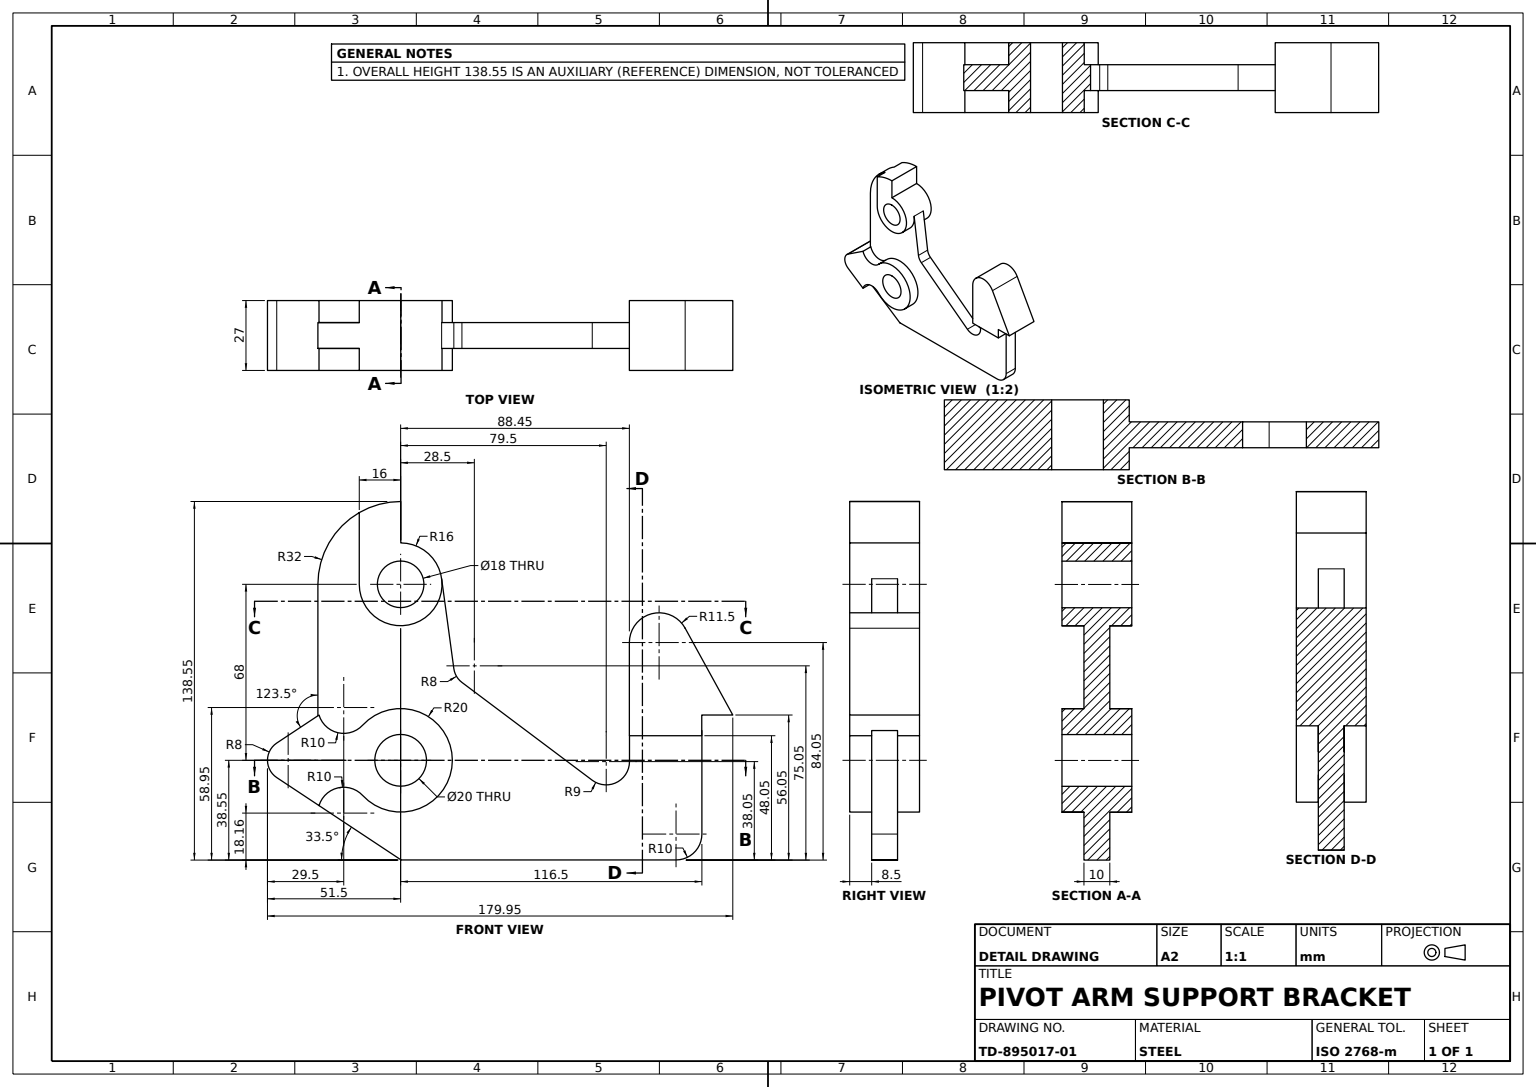
ISO-10303-21;
HEADER;
FILE_DESCRIPTION((''),'2;1');
FILE_NAME('','',(''),(''),'','','');
FILE_SCHEMA(('AUTOMOTIVE_DESIGN'));
ENDSEC;
DATA;
#1=APPLICATION_CONTEXT('');
#2=PRODUCT_CONTEXT('',#1,'mechanical');
#3=PRODUCT('','','',(#2));
#4=PRODUCT_DEFINITION_FORMATION('','',#3);
#5=PRODUCT_DEFINITION_CONTEXT('',#1,'design');
#6=PRODUCT_DEFINITION('','',#4,#5);
#7=PRODUCT_DEFINITION_SHAPE('','',#6);
#8=(LENGTH_UNIT()NAMED_UNIT(*)SI_UNIT(.MILLI.,.METRE.));
#9=(NAMED_UNIT(*)PLANE_ANGLE_UNIT()SI_UNIT($,.RADIAN.));
#10=(NAMED_UNIT(*)SI_UNIT($,.STERADIAN.)SOLID_ANGLE_UNIT());
#11=UNCERTAINTY_MEASURE_WITH_UNIT(LENGTH_MEASURE(0.005),#8,'distance_accuracy_value','');
#12=(GEOMETRIC_REPRESENTATION_CONTEXT(3)GLOBAL_UNCERTAINTY_ASSIGNED_CONTEXT((#11))GLOBAL_UNIT_ASSIGNED_CONTEXT((#8,#9,#10))REPRESENTATION_CONTEXT('',''));
#13=CARTESIAN_POINT('',(-72.916667,-5.,52.097385));
#14=VERTEX_POINT('',#13);
#15=CARTESIAN_POINT('',(-72.916667,-5.,24.902615));
#16=VERTEX_POINT('',#15);
#17=CARTESIAN_POINT('',(-58.25,-5.,38.5));
#18=DIRECTION('',(0.,-1.,0.));
#19=DIRECTION('',(0.,0.,-1.));
#20=AXIS2_PLACEMENT_3D('',#17,#18,#19);
#21=CIRCLE('',#20,20.);
#22=EDGE_CURVE('',#14,#16,#21,.F.);
#23=ORIENTED_EDGE('',*,*,#22,.F.);
#24=CARTESIAN_POINT('',(-72.916667,-13.5,52.097385));
#25=VERTEX_POINT('',#24);
#26=DIRECTION('',(0.,1.,0.));
#27=VECTOR('',#26,1000.);
#28=LINE('',#24,#27);
#29=EDGE_CURVE('',#25,#14,#28,.T.);
#30=ORIENTED_EDGE('',*,*,#29,.F.);
#31=CARTESIAN_POINT('',(-72.916667,-13.5,24.902615));
#32=VERTEX_POINT('',#31);
#33=CARTESIAN_POINT('',(-58.25,-13.5,38.5));
#34=DIRECTION('',(1.,0.,0.));
#35=AXIS2_PLACEMENT_3D('',#33,#18,#34);
#36=CIRCLE('',#35,20.);
#37=EDGE_CURVE('',#32,#25,#36,.T.);
#38=ORIENTED_EDGE('',*,*,#37,.F.);
#39=LINE('',#31,#27);
#40=EDGE_CURVE('',#32,#16,#39,.T.);
#41=ORIENTED_EDGE('',*,*,#40,.T.);
#42=EDGE_LOOP('',(#23,#30,#38,#41));
#43=FACE_BOUND('',#42,.T.);
#44=DIRECTION('',(0.,0.,1.));
#45=AXIS2_PLACEMENT_3D('',#33,#26,#44);
#46=CYLINDRICAL_SURFACE('',#45,20.);
#47=ADVANCED_FACE('',(#43),#46,.T.);
#48=CARTESIAN_POINT('',(-58.2,-13.5,122.499922));
#49=VERTEX_POINT('',#48);
#50=CARTESIAN_POINT('',(-58.2,13.5,122.499922));
#51=VERTEX_POINT('',#50);
#52=LINE('',#48,#27);
#53=EDGE_CURVE('',#49,#51,#52,.T.);
#54=ORIENTED_EDGE('',*,*,#53,.T.);
#55=CARTESIAN_POINT('',(-58.2,13.5,138.499961));
#56=VERTEX_POINT('',#55);
#57=VECTOR('',#19,1000.);
#58=LINE('',#55,#57);
#59=EDGE_CURVE('',#56,#51,#58,.T.);
#60=ORIENTED_EDGE('',*,*,#59,.F.);
#61=CARTESIAN_POINT('',(-58.2,-13.5,138.499961));
#62=VERTEX_POINT('',#61);
#63=LINE('',#61,#27);
#64=EDGE_CURVE('',#62,#56,#63,.T.);
#65=ORIENTED_EDGE('',*,*,#64,.F.);
#66=LINE('',#61,#57);
#67=EDGE_CURVE('',#62,#49,#66,.T.);
#68=ORIENTED_EDGE('',*,*,#67,.T.);
#69=EDGE_LOOP('',(#54,#60,#65,#68));
#70=FACE_BOUND('',#69,.T.);
#71=AXIS2_PLACEMENT_3D('',#61,#34,#19);
#72=PLANE('',#71);
#73=ADVANCED_FACE('',(#70),#72,.T.);
#74=ORIENTED_EDGE('',*,*,#29,.T.);
#75=CARTESIAN_POINT('',(-89.81867,-5.,55.990815));
#76=VERTEX_POINT('',#75);
#77=CARTESIAN_POINT('',(-80.25,-5.,58.896078));
#78=AXIS2_PLACEMENT_3D('',#77,#18,#19);
#79=CIRCLE('',#78,10.);
#80=EDGE_CURVE('',#76,#14,#79,.T.);
#81=ORIENTED_EDGE('',*,*,#80,.F.);
#82=CARTESIAN_POINT('',(-89.81867,-13.5,55.990815));
#83=VERTEX_POINT('',#82);
#84=LINE('',#82,#27);
#85=EDGE_CURVE('',#83,#76,#84,.T.);
#86=ORIENTED_EDGE('',*,*,#85,.F.);
#87=CARTESIAN_POINT('',(-80.25,-13.5,58.896078));
#88=AXIS2_PLACEMENT_3D('',#87,#26,#34);
#89=CIRCLE('',#88,10.);
#90=EDGE_CURVE('',#25,#83,#89,.T.);
#91=ORIENTED_EDGE('',*,*,#90,.F.);
#92=EDGE_LOOP('',(#74,#81,#86,#91));
#93=FACE_BOUND('',#92,.T.);
#94=AXIS2_PLACEMENT_3D('',#87,#26,#44);
#95=CYLINDRICAL_SURFACE('',#94,10.);
#96=ADVANCED_FACE('',(#93),#95,.F.);
#97=CARTESIAN_POINT('',(-58.077253,5.,0.));
#98=VERTEX_POINT('',#97);
#99=CARTESIAN_POINT('',(-58.077253,-5.,0.));
#100=VERTEX_POINT('',#99);
#101=VECTOR('',#18,1000.);
#102=LINE('',#99,#101);
#103=EDGE_CURVE('',#98,#100,#102,.T.);
#104=ORIENTED_EDGE('',*,*,#103,.T.);
#105=CARTESIAN_POINT('',(-58.25,-5.,0.));
#106=VERTEX_POINT('',#105);
#107=CARTESIAN_POINT('',(58.25,-5.,0.));
#108=DIRECTION('',(-1.,0.,0.));
#109=VECTOR('',#108,1000.);
#110=LINE('',#107,#109);
#111=EDGE_CURVE('',#100,#106,#110,.T.);
#112=ORIENTED_EDGE('',*,*,#111,.T.);
#113=CARTESIAN_POINT('',(-58.25,5.,0.));
#114=VERTEX_POINT('',#113);
#115=LINE('',#105,#27);
#116=EDGE_CURVE('',#106,#114,#115,.T.);
#117=ORIENTED_EDGE('',*,*,#116,.T.);
#118=CARTESIAN_POINT('',(58.25,5.,0.));
#119=LINE('',#118,#109);
#120=EDGE_CURVE('',#98,#114,#119,.T.);
#121=ORIENTED_EDGE('',*,*,#120,.F.);
#122=EDGE_LOOP('',(#104,#112,#117,#121));
#123=FACE_BOUND('',#122,.T.);
#124=AXIS2_PLACEMENT_3D('',#107,#19,#108);
#125=PLANE('',#124);
#126=ADVANCED_FACE('',(#123),#125,.T.);
#127=CARTESIAN_POINT('',(58.2,13.5,48.));
#128=VERTEX_POINT('',#127);
#129=CARTESIAN_POINT('',(30.2,13.5,48.));
#130=VERTEX_POINT('',#129);
#131=LINE('',#127,#109);
#132=EDGE_CURVE('',#128,#130,#131,.T.);
#133=ORIENTED_EDGE('',*,*,#132,.T.);
#134=CARTESIAN_POINT('',(30.2,13.5,84.));
#135=VERTEX_POINT('',#134);
#136=VECTOR('',#44,1000.);
#137=LINE('',#129,#136);
#138=EDGE_CURVE('',#130,#135,#137,.T.);
#139=ORIENTED_EDGE('',*,*,#138,.T.);
#140=CARTESIAN_POINT('',(51.779606,13.5,89.536384));
#141=VERTEX_POINT('',#140);
#142=CARTESIAN_POINT('',(41.7,13.5,84.));
#143=AXIS2_PLACEMENT_3D('',#142,#26,#34);
#144=CIRCLE('',#143,11.5);
#145=EDGE_CURVE('',#135,#141,#144,.T.);
#146=ORIENTED_EDGE('',*,*,#145,.T.);
#147=CARTESIAN_POINT('',(70.2,13.5,56.));
#148=VERTEX_POINT('',#147);
#149=DIRECTION('',(0.48142472,0.,-0.876487444));
#150=VECTOR('',#149,1000.);
#151=LINE('',#140,#150);
#152=EDGE_CURVE('',#141,#148,#151,.T.);
#153=ORIENTED_EDGE('',*,*,#152,.T.);
#154=CARTESIAN_POINT('',(58.2,13.5,56.));
#155=VERTEX_POINT('',#154);
#156=LINE('',#147,#109);
#157=EDGE_CURVE('',#148,#155,#156,.T.);
#158=ORIENTED_EDGE('',*,*,#157,.T.);
#159=LINE('',#154,#57);
#160=EDGE_CURVE('',#155,#128,#159,.T.);
#161=ORIENTED_EDGE('',*,*,#160,.T.);
#162=EDGE_LOOP('',(#133,#139,#146,#153,#158,#161));
#163=FACE_BOUND('',#162,.T.);
#164=AXIS2_PLACEMENT_3D('',#142,#26,#44);
#165=PLANE('',#164);
#166=ADVANCED_FACE('',(#163),#165,.T.);
#167=CARTESIAN_POINT('',(-81.480227,5.,27.948867));
#168=VERTEX_POINT('',#167);
#169=CARTESIAN_POINT('',(-81.480227,-5.,27.948867));
#170=VERTEX_POINT('',#169);
#171=LINE('',#169,#101);
#172=EDGE_CURVE('',#168,#170,#171,.T.);
#173=ORIENTED_EDGE('',*,*,#172,.F.);
#174=CARTESIAN_POINT('',(-82.004153,5.,27.948867));
#175=VERTEX_POINT('',#174);
#176=CARTESIAN_POINT('',(-58.,5.,27.948867));
#177=LINE('',#176,#109);
#178=EDGE_CURVE('',#168,#175,#177,.T.);
#179=ORIENTED_EDGE('',*,*,#178,.T.);
#180=CARTESIAN_POINT('',(-82.004153,-5.,27.948867));
#181=VERTEX_POINT('',#180);
#182=CARTESIAN_POINT('',(-82.004153,-13.5,27.948867));
#183=LINE('',#182,#27);
#184=EDGE_CURVE('',#175,#181,#183,.F.);
#185=ORIENTED_EDGE('',*,*,#184,.T.);
#186=CARTESIAN_POINT('',(-58.,-5.,27.948867));
#187=LINE('',#186,#109);
#188=EDGE_CURVE('',#170,#181,#187,.T.);
#189=ORIENTED_EDGE('',*,*,#188,.F.);
#190=EDGE_LOOP('',(#173,#179,#185,#189));
#191=FACE_BOUND('',#190,.T.);
#192=AXIS2_PLACEMENT_3D('',#186,#19,#108);
#193=PLANE('',#192);
#194=ADVANCED_FACE('',(#191),#193,.F.);
#195=CARTESIAN_POINT('',(-58.461253,-5.,0.254164));
#196=VERTEX_POINT('',#195);
#197=DIRECTION('',(-0.639201497,0.,0.769039301));
#198=VECTOR('',#197,1000.);
#199=LINE('',#105,#198);
#200=EDGE_CURVE('',#106,#196,#199,.T.);
#201=ORIENTED_EDGE('',*,*,#200,.T.);
#202=CARTESIAN_POINT('',(-58.461253,5.,0.254164));
#203=VERTEX_POINT('',#202);
#204=LINE('',#195,#27);
#205=EDGE_CURVE('',#196,#203,#204,.T.);
#206=ORIENTED_EDGE('',*,*,#205,.T.);
#207=LINE('',#113,#198);
#208=EDGE_CURVE('',#114,#203,#207,.T.);
#209=ORIENTED_EDGE('',*,*,#208,.F.);
#210=ORIENTED_EDGE('',*,*,#116,.F.);
#211=EDGE_LOOP('',(#201,#206,#209,#210));
#212=FACE_BOUND('',#211,.T.);
#213=DIRECTION('',(-0.769039301,0.,-0.639201497));
#214=AXIS2_PLACEMENT_3D('',#105,#213,#197);
#215=PLANE('',#214);
#216=ADVANCED_FACE('',(#212),#215,.T.);
#217=CARTESIAN_POINT('',(15.85,-5.,30.8));
#218=VERTEX_POINT('',#217);
#219=CARTESIAN_POINT('',(30.25,-5.,38.));
#220=VERTEX_POINT('',#219);
#221=CARTESIAN_POINT('',(21.25,-5.,38.));
#222=AXIS2_PLACEMENT_3D('',#221,#18,#34);
#223=CIRCLE('',#222,9.);
#224=EDGE_CURVE('',#218,#220,#223,.T.);
#225=ORIENTED_EDGE('',*,*,#224,.T.);
#226=CARTESIAN_POINT('',(30.25,5.,38.));
#227=VERTEX_POINT('',#226);
#228=LINE('',#219,#27);
#229=EDGE_CURVE('',#220,#227,#228,.T.);
#230=ORIENTED_EDGE('',*,*,#229,.T.);
#231=CARTESIAN_POINT('',(15.85,5.,30.8));
#232=VERTEX_POINT('',#231);
#233=CARTESIAN_POINT('',(21.25,5.,38.));
#234=AXIS2_PLACEMENT_3D('',#233,#18,#34);
#235=CIRCLE('',#234,9.);
#236=EDGE_CURVE('',#232,#227,#235,.T.);
#237=ORIENTED_EDGE('',*,*,#236,.F.);
#238=LINE('',#217,#27);
#239=EDGE_CURVE('',#218,#232,#238,.T.);
#240=ORIENTED_EDGE('',*,*,#239,.F.);
#241=EDGE_LOOP('',(#225,#230,#237,#240));
#242=FACE_BOUND('',#241,.T.);
#243=AXIS2_PLACEMENT_3D('',#221,#26,#44);
#244=CYLINDRICAL_SURFACE('',#243,9.);
#245=ADVANCED_FACE('',(#242),#244,.F.);
#246=CARTESIAN_POINT('',(30.2,-13.5,84.));
#247=VERTEX_POINT('',#246);
#248=CARTESIAN_POINT('',(51.779606,-13.5,89.536384));
#249=VERTEX_POINT('',#248);
#250=CARTESIAN_POINT('',(41.7,-13.5,84.));
#251=AXIS2_PLACEMENT_3D('',#250,#26,#34);
#252=CIRCLE('',#251,11.5);
#253=EDGE_CURVE('',#247,#249,#252,.T.);
#254=ORIENTED_EDGE('',*,*,#253,.T.);
#255=LINE('',#248,#27);
#256=EDGE_CURVE('',#249,#141,#255,.T.);
#257=ORIENTED_EDGE('',*,*,#256,.T.);
#258=ORIENTED_EDGE('',*,*,#145,.F.);
#259=LINE('',#246,#27);
#260=EDGE_CURVE('',#247,#135,#259,.T.);
#261=ORIENTED_EDGE('',*,*,#260,.F.);
#262=EDGE_LOOP('',(#254,#257,#258,#261));
#263=FACE_BOUND('',#262,.T.);
#264=AXIS2_PLACEMENT_3D('',#250,#26,#44);
#265=CYLINDRICAL_SURFACE('',#264,11.5);
#266=ADVANCED_FACE('',(#263),#265,.T.);
#267=CARTESIAN_POINT('',(-72.916667,5.,52.097385));
#268=VERTEX_POINT('',#267);
#269=CARTESIAN_POINT('',(-72.916667,13.5,52.097385));
#270=VERTEX_POINT('',#269);
#271=EDGE_CURVE('',#268,#270,#28,.T.);
#272=ORIENTED_EDGE('',*,*,#271,.F.);
#273=CARTESIAN_POINT('',(-72.916667,5.,24.902615));
#274=VERTEX_POINT('',#273);
#275=CARTESIAN_POINT('',(-58.25,5.,38.5));
#276=AXIS2_PLACEMENT_3D('',#275,#18,#19);
#277=CIRCLE('',#276,20.);
#278=EDGE_CURVE('',#268,#274,#277,.F.);
#279=ORIENTED_EDGE('',*,*,#278,.T.);
#280=CARTESIAN_POINT('',(-72.916667,13.5,24.902615));
#281=VERTEX_POINT('',#280);
#282=EDGE_CURVE('',#274,#281,#39,.T.);
#283=ORIENTED_EDGE('',*,*,#282,.T.);
#284=CARTESIAN_POINT('',(-58.25,13.5,38.5));
#285=AXIS2_PLACEMENT_3D('',#284,#18,#34);
#286=CIRCLE('',#285,20.);
#287=EDGE_CURVE('',#281,#270,#286,.T.);
#288=ORIENTED_EDGE('',*,*,#287,.T.);
#289=EDGE_LOOP('',(#272,#279,#283,#288));
#290=FACE_BOUND('',#289,.T.);
#291=ADVANCED_FACE('',(#290),#46,.T.);
#292=CARTESIAN_POINT('',(-89.81867,5.,55.990815));
#293=VERTEX_POINT('',#292);
#294=CARTESIAN_POINT('',(-80.25,5.,58.896078));
#295=AXIS2_PLACEMENT_3D('',#294,#18,#19);
#296=CIRCLE('',#295,10.);
#297=EDGE_CURVE('',#293,#268,#296,.T.);
#298=ORIENTED_EDGE('',*,*,#297,.T.);
#299=ORIENTED_EDGE('',*,*,#271,.T.);
#300=CARTESIAN_POINT('',(-89.81867,13.5,55.990815));
#301=VERTEX_POINT('',#300);
#302=CARTESIAN_POINT('',(-80.25,13.5,58.896078));
#303=AXIS2_PLACEMENT_3D('',#302,#26,#34);
#304=CIRCLE('',#303,10.);
#305=EDGE_CURVE('',#270,#301,#304,.T.);
#306=ORIENTED_EDGE('',*,*,#305,.T.);
#307=EDGE_CURVE('',#293,#301,#84,.T.);
#308=ORIENTED_EDGE('',*,*,#307,.F.);
#309=EDGE_LOOP('',(#298,#299,#306,#308));
#310=FACE_BOUND('',#309,.T.);
#311=ADVANCED_FACE('',(#310),#95,.F.);
#312=CARTESIAN_POINT('',(70.2,-13.5,56.));
#313=VERTEX_POINT('',#312);
#314=CARTESIAN_POINT('',(58.2,-13.5,56.));
#315=VERTEX_POINT('',#314);
#316=LINE('',#312,#109);
#317=EDGE_CURVE('',#313,#315,#316,.T.);
#318=ORIENTED_EDGE('',*,*,#317,.T.);
#319=LINE('',#314,#27);
#320=EDGE_CURVE('',#315,#155,#319,.T.);
#321=ORIENTED_EDGE('',*,*,#320,.T.);
#322=ORIENTED_EDGE('',*,*,#157,.F.);
#323=LINE('',#312,#27);
#324=EDGE_CURVE('',#313,#148,#323,.T.);
#325=ORIENTED_EDGE('',*,*,#324,.F.);
#326=EDGE_LOOP('',(#318,#321,#322,#325));
#327=FACE_BOUND('',#326,.T.);
#328=AXIS2_PLACEMENT_3D('',#312,#19,#108);
#329=PLANE('',#328);
#330=ADVANCED_FACE('',(#327),#329,.T.);
#331=CARTESIAN_POINT('',(-74.25,13.5,134.212813));
#332=VERTEX_POINT('',#331);
#333=CARTESIAN_POINT('',(-58.25,13.5,106.5));
#334=AXIS2_PLACEMENT_3D('',#333,#26,#34);
#335=CIRCLE('',#334,32.);
#336=EDGE_CURVE('',#332,#56,#335,.T.);
#337=ORIENTED_EDGE('',*,*,#336,.F.);
#338=CARTESIAN_POINT('',(-74.25,5.,134.212813));
#339=VERTEX_POINT('',#338);
#340=CARTESIAN_POINT('',(-74.25,-13.5,134.212813));
#341=LINE('',#340,#27);
#342=EDGE_CURVE('',#339,#332,#341,.T.);
#343=ORIENTED_EDGE('',*,*,#342,.F.);
#344=CARTESIAN_POINT('',(-90.25,5.,106.5));
#345=VERTEX_POINT('',#344);
#346=CARTESIAN_POINT('',(-58.25,5.,106.5));
#347=AXIS2_PLACEMENT_3D('',#346,#26,#34);
#348=CIRCLE('',#347,32.);
#349=EDGE_CURVE('',#345,#339,#348,.T.);
#350=ORIENTED_EDGE('',*,*,#349,.F.);
#351=CARTESIAN_POINT('',(-90.25,-5.,106.5));
#352=VERTEX_POINT('',#351);
#353=LINE('',#351,#27);
#354=EDGE_CURVE('',#352,#345,#353,.T.);
#355=ORIENTED_EDGE('',*,*,#354,.F.);
#356=CARTESIAN_POINT('',(-74.25,-5.,134.212813));
#357=VERTEX_POINT('',#356);
#358=CARTESIAN_POINT('',(-58.25,-5.,106.5));
#359=AXIS2_PLACEMENT_3D('',#358,#26,#34);
#360=CIRCLE('',#359,32.);
#361=EDGE_CURVE('',#352,#357,#360,.T.);
#362=ORIENTED_EDGE('',*,*,#361,.T.);
#363=VERTEX_POINT('',#340);
#364=EDGE_CURVE('',#363,#357,#341,.T.);
#365=ORIENTED_EDGE('',*,*,#364,.F.);
#366=CARTESIAN_POINT('',(-58.25,-13.5,106.5));
#367=AXIS2_PLACEMENT_3D('',#366,#26,#34);
#368=CIRCLE('',#367,32.);
#369=EDGE_CURVE('',#363,#62,#368,.T.);
#370=ORIENTED_EDGE('',*,*,#369,.T.);
#371=ORIENTED_EDGE('',*,*,#64,.T.);
#372=EDGE_LOOP('',(#337,#343,#350,#355,#362,#365,#370,#371));
#373=FACE_BOUND('',#372,.T.);
#374=AXIS2_PLACEMENT_3D('',#358,#26,#44);
#375=CYLINDRICAL_SURFACE('',#374,32.);
#376=ADVANCED_FACE('',(#373),#375,.T.);
#377=CARTESIAN_POINT('',(-34.55,-5.,68.6));
#378=VERTEX_POINT('',#377);
#379=CARTESIAN_POINT('',(-34.55,5.,68.6));
#380=VERTEX_POINT('',#379);
#381=LINE('',#377,#27);
#382=EDGE_CURVE('',#378,#380,#381,.T.);
#383=ORIENTED_EDGE('',*,*,#382,.F.);
#384=DIRECTION('',(0.8,0.,-0.6));
#385=VECTOR('',#384,1000.);
#386=LINE('',#377,#385);
#387=EDGE_CURVE('',#378,#218,#386,.T.);
#388=ORIENTED_EDGE('',*,*,#387,.T.);
#389=ORIENTED_EDGE('',*,*,#239,.T.);
#390=LINE('',#379,#385);
#391=EDGE_CURVE('',#380,#232,#390,.T.);
#392=ORIENTED_EDGE('',*,*,#391,.F.);
#393=EDGE_LOOP('',(#383,#388,#389,#392));
#394=FACE_BOUND('',#393,.T.);
#395=DIRECTION('',(0.6,0.,0.8));
#396=AXIS2_PLACEMENT_3D('',#377,#395,#384);
#397=PLANE('',#396);
#398=ADVANCED_FACE('',(#394),#397,.T.);
#399=CARTESIAN_POINT('',(-58.25,13.5,115.5));
#400=VERTEX_POINT('',#399);
#401=AXIS2_PLACEMENT_3D('',#333,#26,#44);
#402=CIRCLE('',#401,9.);
#403=EDGE_CURVE('',#400,#400,#402,.T.);
#404=ORIENTED_EDGE('',*,*,#403,.T.);
#405=EDGE_LOOP('',(#404));
#406=FACE_BOUND('',#405,.T.);
#407=CARTESIAN_POINT('',(-58.25,-13.5,115.5));
#408=VERTEX_POINT('',#407);
#409=AXIS2_PLACEMENT_3D('',#366,#26,#44);
#410=CIRCLE('',#409,9.);
#411=EDGE_CURVE('',#408,#408,#410,.T.);
#412=ORIENTED_EDGE('',*,*,#411,.F.);
#413=EDGE_LOOP('',(#412));
#414=FACE_BOUND('',#413,.T.);
#415=CYLINDRICAL_SURFACE('',#409,9.);
#416=ADVANCED_FACE('',(#406,#414),#415,.F.);
#417=CARTESIAN_POINT('',(58.25,-5.,10.));
#418=VERTEX_POINT('',#417);
#419=CARTESIAN_POINT('',(58.25,5.,10.));
#420=VERTEX_POINT('',#419);
#421=LINE('',#417,#27);
#422=EDGE_CURVE('',#418,#420,#421,.T.);
#423=ORIENTED_EDGE('',*,*,#422,.F.);
#424=CARTESIAN_POINT('',(48.25,-5.,0.));
#425=VERTEX_POINT('',#424);
#426=CARTESIAN_POINT('',(48.25,-5.,10.));
#427=AXIS2_PLACEMENT_3D('',#426,#18,#19);
#428=CIRCLE('',#427,10.);
#429=EDGE_CURVE('',#425,#418,#428,.T.);
#430=ORIENTED_EDGE('',*,*,#429,.F.);
#431=CARTESIAN_POINT('',(48.25,5.,0.));
#432=VERTEX_POINT('',#431);
#433=LINE('',#424,#27);
#434=EDGE_CURVE('',#432,#425,#433,.F.);
#435=ORIENTED_EDGE('',*,*,#434,.F.);
#436=CARTESIAN_POINT('',(48.25,5.,10.));
#437=AXIS2_PLACEMENT_3D('',#436,#18,#19);
#438=CIRCLE('',#437,10.);
#439=EDGE_CURVE('',#420,#432,#438,.F.);
#440=ORIENTED_EDGE('',*,*,#439,.F.);
#441=EDGE_LOOP('',(#423,#430,#435,#440));
#442=FACE_BOUND('',#441,.T.);
#443=AXIS2_PLACEMENT_3D('',#426,#26,#44);
#444=CYLINDRICAL_SURFACE('',#443,10.);
#445=ADVANCED_FACE('',(#442),#444,.T.);
#446=CARTESIAN_POINT('',(-74.25,-13.5,106.5));
#447=VERTEX_POINT('',#446);
#448=LINE('',#446,#136);
#449=EDGE_CURVE('',#447,#363,#448,.T.);
#450=ORIENTED_EDGE('',*,*,#449,.F.);
#451=CIRCLE('',#367,16.);
#452=EDGE_CURVE('',#49,#447,#451,.T.);
#453=ORIENTED_EDGE('',*,*,#452,.F.);
#454=ORIENTED_EDGE('',*,*,#67,.F.);
#455=ORIENTED_EDGE('',*,*,#369,.F.);
#456=EDGE_LOOP('',(#450,#453,#454,#455));
#457=FACE_BOUND('',#456,.T.);
#458=ORIENTED_EDGE('',*,*,#411,.T.);
#459=EDGE_LOOP('',(#458));
#460=FACE_BOUND('',#459,.T.);
#461=PLANE('',#409);
#462=ADVANCED_FACE('',(#457,#460),#461,.F.);
#463=CARTESIAN_POINT('',(-74.25,-5.,106.5));
#464=VERTEX_POINT('',#463);
#465=CARTESIAN_POINT('',(-74.25,-5.,38.));
#466=LINE('',#465,#57);
#467=EDGE_CURVE('',#357,#464,#466,.T.);
#468=ORIENTED_EDGE('',*,*,#467,.T.);
#469=LINE('',#446,#27);
#470=EDGE_CURVE('',#447,#464,#469,.T.);
#471=ORIENTED_EDGE('',*,*,#470,.F.);
#472=ORIENTED_EDGE('',*,*,#449,.T.);
#473=ORIENTED_EDGE('',*,*,#364,.T.);
#474=EDGE_LOOP('',(#468,#471,#472,#473));
#475=FACE_BOUND('',#474,.T.);
#476=AXIS2_PLACEMENT_3D('',#446,#108,#44);
#477=PLANE('',#476);
#478=ADVANCED_FACE('',(#475),#477,.T.);
#479=CARTESIAN_POINT('',(30.25,5.,48.));
#480=VERTEX_POINT('',#479);
#481=CARTESIAN_POINT('',(30.25,-5.,48.));
#482=VERTEX_POINT('',#481);
#483=LINE('',#481,#101);
#484=EDGE_CURVE('',#480,#482,#483,.T.);
#485=ORIENTED_EDGE('',*,*,#484,.F.);
#486=LINE('',#226,#136);
#487=EDGE_CURVE('',#227,#480,#486,.T.);
#488=ORIENTED_EDGE('',*,*,#487,.F.);
#489=ORIENTED_EDGE('',*,*,#229,.F.);
#490=LINE('',#219,#136);
#491=EDGE_CURVE('',#220,#482,#490,.T.);
#492=ORIENTED_EDGE('',*,*,#491,.T.);
#493=EDGE_LOOP('',(#485,#488,#489,#492));
#494=FACE_BOUND('',#493,.T.);
#495=AXIS2_PLACEMENT_3D('',#219,#108,#44);
#496=PLANE('',#495);
#497=ADVANCED_FACE('',(#494),#496,.T.);
#498=CARTESIAN_POINT('',(-89.81867,5.,21.009185));
#499=VERTEX_POINT('',#498);
#500=CARTESIAN_POINT('',(-100.303385,5.,27.948867));
#501=DIRECTION('',(0.833885822,0.,-0.551936985));
#502=VECTOR('',#501,1000.);
#503=LINE('',#500,#502);
#504=EDGE_CURVE('',#499,#203,#503,.T.);
#505=ORIENTED_EDGE('',*,*,#504,.T.);
#506=ORIENTED_EDGE('',*,*,#205,.F.);
#507=CARTESIAN_POINT('',(-89.81867,-5.,21.009185));
#508=VERTEX_POINT('',#507);
#509=CARTESIAN_POINT('',(-100.303385,-5.,27.948867));
#510=LINE('',#509,#502);
#511=EDGE_CURVE('',#508,#196,#510,.T.);
#512=ORIENTED_EDGE('',*,*,#511,.F.);
#513=CARTESIAN_POINT('',(-89.81867,-13.5,21.009185));
#514=VERTEX_POINT('',#513);
#515=LINE('',#513,#27);
#516=EDGE_CURVE('',#514,#508,#515,.T.);
#517=ORIENTED_EDGE('',*,*,#516,.F.);
#518=CARTESIAN_POINT('',(-106.165496,-13.5,31.828913));
#519=VERTEX_POINT('',#518);
#520=LINE('',#518,#502);
#521=EDGE_CURVE('',#519,#514,#520,.T.);
#522=ORIENTED_EDGE('',*,*,#521,.F.);
#523=CARTESIAN_POINT('',(-106.165496,13.5,31.828913));
#524=VERTEX_POINT('',#523);
#525=LINE('',#518,#27);
#526=EDGE_CURVE('',#519,#524,#525,.T.);
#527=ORIENTED_EDGE('',*,*,#526,.T.);
#528=CARTESIAN_POINT('',(-89.81867,13.5,21.009185));
#529=VERTEX_POINT('',#528);
#530=LINE('',#523,#502);
#531=EDGE_CURVE('',#524,#529,#530,.T.);
#532=ORIENTED_EDGE('',*,*,#531,.T.);
#533=EDGE_CURVE('',#499,#529,#515,.T.);
#534=ORIENTED_EDGE('',*,*,#533,.F.);
#535=EDGE_LOOP('',(#505,#506,#512,#517,#522,#527,#532,#534));
#536=FACE_BOUND('',#535,.T.);
#537=DIRECTION('',(0.551936985,0.,0.833885822));
#538=AXIS2_PLACEMENT_3D('',#518,#537,#501);
#539=PLANE('',#538);
#540=ADVANCED_FACE('',(#536),#539,.F.);
#541=CARTESIAN_POINT('',(58.2,-5.,48.));
#542=VERTEX_POINT('',#541);
#543=CARTESIAN_POINT('',(58.2,-5.,50.));
#544=VERTEX_POINT('',#543);
#545=CARTESIAN_POINT('',(58.2,-5.,38.));
#546=LINE('',#545,#136);
#547=EDGE_CURVE('',#542,#544,#546,.T.);
#548=ORIENTED_EDGE('',*,*,#547,.T.);
#549=CARTESIAN_POINT('',(58.2,5.,50.));
#550=VERTEX_POINT('',#549);
#551=LINE('',#543,#27);
#552=EDGE_CURVE('',#544,#550,#551,.T.);
#553=ORIENTED_EDGE('',*,*,#552,.T.);
#554=CARTESIAN_POINT('',(58.2,5.,48.));
#555=VERTEX_POINT('',#554);
#556=CARTESIAN_POINT('',(58.2,5.,38.));
#557=LINE('',#556,#136);
#558=EDGE_CURVE('',#555,#550,#557,.T.);
#559=ORIENTED_EDGE('',*,*,#558,.F.);
#560=CARTESIAN_POINT('',(58.2,-13.5,48.));
#561=LINE('',#560,#27);
#562=EDGE_CURVE('',#555,#128,#561,.T.);
#563=ORIENTED_EDGE('',*,*,#562,.T.);
#564=ORIENTED_EDGE('',*,*,#160,.F.);
#565=ORIENTED_EDGE('',*,*,#320,.F.);
#566=VERTEX_POINT('',#560);
#567=LINE('',#314,#57);
#568=EDGE_CURVE('',#315,#566,#567,.T.);
#569=ORIENTED_EDGE('',*,*,#568,.T.);
#570=EDGE_CURVE('',#566,#542,#561,.T.);
#571=ORIENTED_EDGE('',*,*,#570,.T.);
#572=EDGE_LOOP('',(#548,#553,#559,#563,#564,#565,#569,#571));
#573=FACE_BOUND('',#572,.T.);
#574=AXIS2_PLACEMENT_3D('',#314,#34,#19);
#575=PLANE('',#574);
#576=ADVANCED_FACE('',(#573),#575,.T.);
#577=CARTESIAN_POINT('',(30.2,-13.5,48.));
#578=VERTEX_POINT('',#577);
#579=LINE('',#577,#27);
#580=EDGE_CURVE('',#578,#130,#579,.T.);
#581=ORIENTED_EDGE('',*,*,#580,.F.);
#582=LINE('',#577,#136);
#583=EDGE_CURVE('',#578,#247,#582,.T.);
#584=ORIENTED_EDGE('',*,*,#583,.T.);
#585=ORIENTED_EDGE('',*,*,#260,.T.);
#586=ORIENTED_EDGE('',*,*,#138,.F.);
#587=EDGE_LOOP('',(#581,#584,#585,#586));
#588=FACE_BOUND('',#587,.T.);
#589=AXIS2_PLACEMENT_3D('',#577,#108,#44);
#590=PLANE('',#589);
#591=ADVANCED_FACE('',(#588),#590,.T.);
#592=ORIENTED_EDGE('',*,*,#256,.F.);
#593=LINE('',#248,#150);
#594=EDGE_CURVE('',#249,#313,#593,.T.);
#595=ORIENTED_EDGE('',*,*,#594,.T.);
#596=ORIENTED_EDGE('',*,*,#324,.T.);
#597=ORIENTED_EDGE('',*,*,#152,.F.);
#598=EDGE_LOOP('',(#592,#595,#596,#597));
#599=FACE_BOUND('',#598,.T.);
#600=DIRECTION('',(0.876487444,0.,0.48142472));
#601=AXIS2_PLACEMENT_3D('',#248,#600,#149);
#602=PLANE('',#601);
#603=ADVANCED_FACE('',(#599),#602,.T.);
#604=ORIENTED_EDGE('',*,*,#583,.F.);
#605=LINE('',#560,#109);
#606=EDGE_CURVE('',#566,#578,#605,.T.);
#607=ORIENTED_EDGE('',*,*,#606,.F.);
#608=ORIENTED_EDGE('',*,*,#568,.F.);
#609=ORIENTED_EDGE('',*,*,#317,.F.);
#610=ORIENTED_EDGE('',*,*,#594,.F.);
#611=ORIENTED_EDGE('',*,*,#253,.F.);
#612=EDGE_LOOP('',(#604,#607,#608,#609,#610,#611));
#613=FACE_BOUND('',#612,.T.);
#614=PLANE('',#264);
#615=ADVANCED_FACE('',(#613),#614,.F.);
#616=CARTESIAN_POINT('',(-81.53969,-5.,28.020408));
#617=VERTEX_POINT('',#616);
#618=EDGE_CURVE('',#170,#617,#199,.T.);
#619=ORIENTED_EDGE('',*,*,#618,.T.);
#620=CARTESIAN_POINT('',(-81.53969,5.,28.020408));
#621=VERTEX_POINT('',#620);
#622=CARTESIAN_POINT('',(-81.53969,-13.5,28.020408));
#623=LINE('',#622,#27);
#624=EDGE_CURVE('',#617,#621,#623,.T.);
#625=ORIENTED_EDGE('',*,*,#624,.T.);
#626=EDGE_CURVE('',#168,#621,#207,.T.);
#627=ORIENTED_EDGE('',*,*,#626,.F.);
#628=ORIENTED_EDGE('',*,*,#172,.T.);
#629=EDGE_LOOP('',(#619,#625,#627,#628));
#630=FACE_BOUND('',#629,.T.);
#631=ADVANCED_FACE('',(#630),#215,.T.);
#632=CARTESIAN_POINT('',(-37.677177,-5.,73.92303));
#633=VERTEX_POINT('',#632);
#634=CARTESIAN_POINT('',(-37.677177,5.,73.92303));
#635=VERTEX_POINT('',#634);
#636=LINE('',#632,#27);
#637=EDGE_CURVE('',#633,#635,#636,.T.);
#638=ORIENTED_EDGE('',*,*,#637,.T.);
#639=CARTESIAN_POINT('',(-42.395646,5.,108.653939));
#640=VERTEX_POINT('',#639);
#641=DIRECTION('',(0.134621216,0.,-0.990897133));
#642=VECTOR('',#641,1000.);
#643=LINE('',#639,#642);
#644=EDGE_CURVE('',#640,#635,#643,.T.);
#645=ORIENTED_EDGE('',*,*,#644,.F.);
#646=CARTESIAN_POINT('',(-42.395646,-5.,108.653939));
#647=VERTEX_POINT('',#646);
#648=LINE('',#646,#27);
#649=EDGE_CURVE('',#647,#640,#648,.T.);
#650=ORIENTED_EDGE('',*,*,#649,.F.);
#651=LINE('',#646,#642);
#652=EDGE_CURVE('',#647,#633,#651,.T.);
#653=ORIENTED_EDGE('',*,*,#652,.T.);
#654=EDGE_LOOP('',(#638,#645,#650,#653));
#655=FACE_BOUND('',#654,.T.);
#656=DIRECTION('',(0.990897133,0.,0.134621216));
#657=AXIS2_PLACEMENT_3D('',#646,#656,#641);
#658=PLANE('',#657);
#659=ADVANCED_FACE('',(#655),#658,.T.);
#660=CARTESIAN_POINT('',(-58.,-5.,-0.051133));
#661=VERTEX_POINT('',#660);
#662=CARTESIAN_POINT('',(-58.,5.,-0.051133));
#663=VERTEX_POINT('',#662);
#664=LINE('',#660,#27);
#665=EDGE_CURVE('',#661,#663,#664,.T.);
#666=ORIENTED_EDGE('',*,*,#665,.F.);
#667=EDGE_CURVE('',#100,#661,#510,.T.);
#668=ORIENTED_EDGE('',*,*,#667,.F.);
#669=ORIENTED_EDGE('',*,*,#103,.F.);
#670=EDGE_CURVE('',#98,#663,#503,.T.);
#671=ORIENTED_EDGE('',*,*,#670,.T.);
#672=EDGE_LOOP('',(#666,#668,#669,#671));
#673=FACE_BOUND('',#672,.T.);
#674=AXIS2_PLACEMENT_3D('',#509,#537,#501);
#675=PLANE('',#674);
#676=ADVANCED_FACE('',(#673),#675,.F.);
#677=ORIENTED_EDGE('',*,*,#624,.F.);
#678=CARTESIAN_POINT('',(-80.25,-5.,18.103922));
#679=AXIS2_PLACEMENT_3D('',#678,#18,#19);
#680=CIRCLE('',#679,10.);
#681=EDGE_CURVE('',#16,#617,#680,.T.);
#682=ORIENTED_EDGE('',*,*,#681,.F.);
#683=ORIENTED_EDGE('',*,*,#40,.F.);
#684=CARTESIAN_POINT('',(-80.25,-13.5,18.103922));
#685=AXIS2_PLACEMENT_3D('',#684,#26,#34);
#686=CIRCLE('',#685,10.);
#687=EDGE_CURVE('',#514,#32,#686,.T.);
#688=ORIENTED_EDGE('',*,*,#687,.F.);
#689=ORIENTED_EDGE('',*,*,#516,.T.);
#690=EDGE_CURVE('',#181,#508,#680,.T.);
#691=ORIENTED_EDGE('',*,*,#690,.F.);
#692=ORIENTED_EDGE('',*,*,#184,.F.);
#693=CARTESIAN_POINT('',(-80.25,5.,18.103922));
#694=AXIS2_PLACEMENT_3D('',#693,#18,#19);
#695=CIRCLE('',#694,10.);
#696=EDGE_CURVE('',#175,#499,#695,.T.);
#697=ORIENTED_EDGE('',*,*,#696,.T.);
#698=ORIENTED_EDGE('',*,*,#533,.T.);
#699=CARTESIAN_POINT('',(-80.25,13.5,18.103922));
#700=AXIS2_PLACEMENT_3D('',#699,#26,#34);
#701=CIRCLE('',#700,10.);
#702=EDGE_CURVE('',#529,#281,#701,.T.);
#703=ORIENTED_EDGE('',*,*,#702,.T.);
#704=ORIENTED_EDGE('',*,*,#282,.F.);
#705=EDGE_CURVE('',#274,#621,#695,.T.);
#706=ORIENTED_EDGE('',*,*,#705,.T.);
#707=EDGE_LOOP('',(#677,#682,#683,#688,#689,#691,#692,#697,#698,#703,#704,#706));
#708=FACE_BOUND('',#707,.T.);
#709=AXIS2_PLACEMENT_3D('',#684,#26,#44);
#710=CYLINDRICAL_SURFACE('',#709,10.);
#711=ADVANCED_FACE('',(#708),#710,.F.);
#712=CARTESIAN_POINT('',(-90.25,5.,55.705324));
#713=VERTEX_POINT('',#712);
#714=CARTESIAN_POINT('',(-90.25,5.,38.5));
#715=LINE('',#714,#136);
#716=EDGE_CURVE('',#713,#345,#715,.T.);
#717=ORIENTED_EDGE('',*,*,#716,.T.);
#718=ORIENTED_EDGE('',*,*,#349,.T.);
#719=CARTESIAN_POINT('',(-74.25,5.,106.5));
#720=VERTEX_POINT('',#719);
#721=CARTESIAN_POINT('',(-74.25,5.,38.));
#722=LINE('',#721,#57);
#723=EDGE_CURVE('',#339,#720,#722,.T.);
#724=ORIENTED_EDGE('',*,*,#723,.T.);
#725=AXIS2_PLACEMENT_3D('',#346,#18,#19);
#726=CIRCLE('',#725,16.);
#727=EDGE_CURVE('',#720,#640,#726,.T.);
#728=ORIENTED_EDGE('',*,*,#727,.T.);
#729=ORIENTED_EDGE('',*,*,#644,.T.);
#730=CARTESIAN_POINT('',(-29.75,5.,75.));
#731=AXIS2_PLACEMENT_3D('',#730,#18,#34);
#732=CIRCLE('',#731,8.);
#733=EDGE_CURVE('',#635,#380,#732,.T.);
#734=ORIENTED_EDGE('',*,*,#733,.T.);
#735=ORIENTED_EDGE('',*,*,#391,.T.);
#736=ORIENTED_EDGE('',*,*,#236,.T.);
#737=ORIENTED_EDGE('',*,*,#487,.T.);
#738=CARTESIAN_POINT('',(21.25,5.,48.));
#739=VECTOR('',#34,1000.);
#740=LINE('',#738,#739);
#741=EDGE_CURVE('',#480,#555,#740,.T.);
#742=ORIENTED_EDGE('',*,*,#741,.T.);
#743=ORIENTED_EDGE('',*,*,#558,.T.);
#744=CARTESIAN_POINT('',(58.25,5.,50.));
#745=VERTEX_POINT('',#744);
#746=CARTESIAN_POINT('',(30.25,5.,50.));
#747=LINE('',#746,#739);
#748=EDGE_CURVE('',#550,#745,#747,.T.);
#749=ORIENTED_EDGE('',*,*,#748,.T.);
#750=LINE('',#744,#57);
#751=EDGE_CURVE('',#745,#420,#750,.T.);
#752=ORIENTED_EDGE('',*,*,#751,.T.);
#753=ORIENTED_EDGE('',*,*,#439,.T.);
#754=CARTESIAN_POINT('',(-58.,5.,0.));
#755=VERTEX_POINT('',#754);
#756=EDGE_CURVE('',#432,#755,#119,.T.);
#757=ORIENTED_EDGE('',*,*,#756,.T.);
#758=LINE('',#662,#136);
#759=EDGE_CURVE('',#663,#755,#758,.T.);
#760=ORIENTED_EDGE('',*,*,#759,.F.);
#761=ORIENTED_EDGE('',*,*,#670,.F.);
#762=ORIENTED_EDGE('',*,*,#120,.T.);
#763=ORIENTED_EDGE('',*,*,#208,.T.);
#764=ORIENTED_EDGE('',*,*,#504,.F.);
#765=ORIENTED_EDGE('',*,*,#696,.F.);
#766=ORIENTED_EDGE('',*,*,#178,.F.);
#767=ORIENTED_EDGE('',*,*,#626,.T.);
#768=ORIENTED_EDGE('',*,*,#705,.F.);
#769=ORIENTED_EDGE('',*,*,#278,.F.);
#770=ORIENTED_EDGE('',*,*,#297,.F.);
#771=CARTESIAN_POINT('',(-20.865658,5.,101.629818));
#772=DIRECTION('',(0.833885822,0.,0.551936985));
#773=VECTOR('',#772,1000.);
#774=LINE('',#771,#773);
#775=EDGE_CURVE('',#713,#293,#774,.T.);
#776=ORIENTED_EDGE('',*,*,#775,.F.);
#777=EDGE_LOOP('',(#717,#718,#724,#728,#729,#734,#735,#736,#737,#742,#743,#749,#752,#753,#757,#760,#761,#762,#763,#764,#765,#766,#767,#768,#769,#770,#776));
#778=FACE_BOUND('',#777,.T.);
#779=AXIS2_PLACEMENT_3D('',#233,#18,#19);
#780=PLANE('',#779);
#781=ADVANCED_FACE('',(#778),#780,.F.);
#782=CARTESIAN_POINT('',(-106.165496,13.5,45.171087));
#783=VERTEX_POINT('',#782);
#784=CARTESIAN_POINT('',(-101.75,13.5,38.5));
#785=AXIS2_PLACEMENT_3D('',#784,#18,#34);
#786=CIRCLE('',#785,8.);
#787=EDGE_CURVE('',#783,#524,#786,.T.);
#788=ORIENTED_EDGE('',*,*,#787,.T.);
#789=ORIENTED_EDGE('',*,*,#526,.F.);
#790=CARTESIAN_POINT('',(-106.165496,-13.5,45.171087));
#791=VERTEX_POINT('',#790);
#792=CARTESIAN_POINT('',(-101.75,-13.5,38.5));
#793=AXIS2_PLACEMENT_3D('',#792,#18,#34);
#794=CIRCLE('',#793,8.);
#795=EDGE_CURVE('',#791,#519,#794,.T.);
#796=ORIENTED_EDGE('',*,*,#795,.F.);
#797=LINE('',#790,#27);
#798=EDGE_CURVE('',#791,#783,#797,.T.);
#799=ORIENTED_EDGE('',*,*,#798,.T.);
#800=EDGE_LOOP('',(#788,#789,#796,#799));
#801=FACE_BOUND('',#800,.T.);
#802=AXIS2_PLACEMENT_3D('',#792,#26,#44);
#803=CYLINDRICAL_SURFACE('',#802,8.);
#804=ADVANCED_FACE('',(#801),#803,.T.);
#805=CARTESIAN_POINT('',(-58.,-5.,0.));
#806=VERTEX_POINT('',#805);
#807=LINE('',#805,#27);
#808=EDGE_CURVE('',#806,#755,#807,.T.);
#809=ORIENTED_EDGE('',*,*,#808,.F.);
#810=LINE('',#660,#136);
#811=EDGE_CURVE('',#661,#806,#810,.T.);
#812=ORIENTED_EDGE('',*,*,#811,.F.);
#813=ORIENTED_EDGE('',*,*,#665,.T.);
#814=ORIENTED_EDGE('',*,*,#759,.T.);
#815=EDGE_LOOP('',(#809,#812,#813,#814));
#816=FACE_BOUND('',#815,.T.);
#817=AXIS2_PLACEMENT_3D('',#660,#108,#44);
#818=PLANE('',#817);
#819=ADVANCED_FACE('',(#816),#818,.F.);
#820=ORIENTED_EDGE('',*,*,#808,.T.);
#821=ORIENTED_EDGE('',*,*,#756,.F.);
#822=ORIENTED_EDGE('',*,*,#434,.T.);
#823=EDGE_CURVE('',#425,#806,#110,.T.);
#824=ORIENTED_EDGE('',*,*,#823,.T.);
#825=EDGE_LOOP('',(#820,#821,#822,#824));
#826=FACE_BOUND('',#825,.T.);
#827=ADVANCED_FACE('',(#826),#125,.T.);
#828=CARTESIAN_POINT('',(-58.25,13.5,28.5));
#829=VERTEX_POINT('',#828);
#830=AXIS2_PLACEMENT_3D('',#284,#18,#19);
#831=CIRCLE('',#830,10.);
#832=EDGE_CURVE('',#829,#829,#831,.T.);
#833=ORIENTED_EDGE('',*,*,#832,.T.);
#834=EDGE_LOOP('',(#833));
#835=FACE_BOUND('',#834,.T.);
#836=ORIENTED_EDGE('',*,*,#702,.F.);
#837=ORIENTED_EDGE('',*,*,#531,.F.);
#838=ORIENTED_EDGE('',*,*,#787,.F.);
#839=DIRECTION('',(-0.833885822,0.,-0.551936985));
#840=VECTOR('',#839,1000.);
#841=LINE('',#300,#840);
#842=EDGE_CURVE('',#301,#783,#841,.T.);
#843=ORIENTED_EDGE('',*,*,#842,.F.);
#844=ORIENTED_EDGE('',*,*,#305,.F.);
#845=ORIENTED_EDGE('',*,*,#287,.F.);
#846=EDGE_LOOP('',(#836,#837,#838,#843,#844,#845));
#847=FACE_BOUND('',#846,.T.);
#848=PLANE('',#830);
#849=ADVANCED_FACE('',(#835,#847),#848,.F.);
#850=CARTESIAN_POINT('',(-58.25,-13.5,48.5));
#851=VERTEX_POINT('',#850);
#852=CIRCLE('',#45,10.);
#853=EDGE_CURVE('',#851,#851,#852,.T.);
#854=ORIENTED_EDGE('',*,*,#853,.T.);
#855=EDGE_LOOP('',(#854));
#856=FACE_BOUND('',#855,.T.);
#857=ORIENTED_EDGE('',*,*,#795,.T.);
#858=ORIENTED_EDGE('',*,*,#521,.T.);
#859=ORIENTED_EDGE('',*,*,#687,.T.);
#860=ORIENTED_EDGE('',*,*,#37,.T.);
#861=ORIENTED_EDGE('',*,*,#90,.T.);
#862=LINE('',#82,#840);
#863=EDGE_CURVE('',#83,#791,#862,.T.);
#864=ORIENTED_EDGE('',*,*,#863,.T.);
#865=EDGE_LOOP('',(#857,#858,#859,#860,#861,#864));
#866=FACE_BOUND('',#865,.T.);
#867=AXIS2_PLACEMENT_3D('',#33,#18,#19);
#868=PLANE('',#867);
#869=ADVANCED_FACE('',(#856,#866),#868,.T.);
#870=ORIENTED_EDGE('',*,*,#552,.F.);
#871=CARTESIAN_POINT('',(58.25,-5.,50.));
#872=VERTEX_POINT('',#871);
#873=CARTESIAN_POINT('',(30.25,-5.,50.));
#874=LINE('',#873,#739);
#875=EDGE_CURVE('',#544,#872,#874,.T.);
#876=ORIENTED_EDGE('',*,*,#875,.T.);
#877=LINE('',#871,#27);
#878=EDGE_CURVE('',#872,#745,#877,.T.);
#879=ORIENTED_EDGE('',*,*,#878,.T.);
#880=ORIENTED_EDGE('',*,*,#748,.F.);
#881=EDGE_LOOP('',(#870,#876,#879,#880));
#882=FACE_BOUND('',#881,.T.);
#883=AXIS2_PLACEMENT_3D('',#873,#44,#34);
#884=PLANE('',#883);
#885=ADVANCED_FACE('',(#882),#884,.T.);
#886=CARTESIAN_POINT('',(-74.25,13.5,106.5));
#887=VERTEX_POINT('',#886);
#888=LINE('',#886,#136);
#889=EDGE_CURVE('',#887,#332,#888,.T.);
#890=ORIENTED_EDGE('',*,*,#889,.F.);
#891=EDGE_CURVE('',#720,#887,#469,.T.);
#892=ORIENTED_EDGE('',*,*,#891,.F.);
#893=ORIENTED_EDGE('',*,*,#723,.F.);
#894=ORIENTED_EDGE('',*,*,#342,.T.);
#895=EDGE_LOOP('',(#890,#892,#893,#894));
#896=FACE_BOUND('',#895,.T.);
#897=ADVANCED_FACE('',(#896),#477,.T.);
#898=ORIENTED_EDGE('',*,*,#832,.F.);
#899=EDGE_LOOP('',(#898));
#900=FACE_BOUND('',#899,.T.);
#901=ORIENTED_EDGE('',*,*,#853,.F.);
#902=EDGE_LOOP('',(#901));
#903=FACE_BOUND('',#902,.T.);
#904=CYLINDRICAL_SURFACE('',#45,10.);
#905=ADVANCED_FACE('',(#900,#903),#904,.F.);
#906=ORIENTED_EDGE('',*,*,#690,.T.);
#907=ORIENTED_EDGE('',*,*,#511,.T.);
#908=ORIENTED_EDGE('',*,*,#200,.F.);
#909=ORIENTED_EDGE('',*,*,#111,.F.);
#910=ORIENTED_EDGE('',*,*,#667,.T.);
#911=ORIENTED_EDGE('',*,*,#811,.T.);
#912=ORIENTED_EDGE('',*,*,#823,.F.);
#913=ORIENTED_EDGE('',*,*,#429,.T.);
#914=LINE('',#871,#57);
#915=EDGE_CURVE('',#872,#418,#914,.T.);
#916=ORIENTED_EDGE('',*,*,#915,.F.);
#917=ORIENTED_EDGE('',*,*,#875,.F.);
#918=ORIENTED_EDGE('',*,*,#547,.F.);
#919=CARTESIAN_POINT('',(21.25,-5.,48.));
#920=LINE('',#919,#739);
#921=EDGE_CURVE('',#482,#542,#920,.T.);
#922=ORIENTED_EDGE('',*,*,#921,.F.);
#923=ORIENTED_EDGE('',*,*,#491,.F.);
#924=ORIENTED_EDGE('',*,*,#224,.F.);
#925=ORIENTED_EDGE('',*,*,#387,.F.);
#926=CARTESIAN_POINT('',(-29.75,-5.,75.));
#927=AXIS2_PLACEMENT_3D('',#926,#18,#34);
#928=CIRCLE('',#927,8.);
#929=EDGE_CURVE('',#633,#378,#928,.T.);
#930=ORIENTED_EDGE('',*,*,#929,.F.);
#931=ORIENTED_EDGE('',*,*,#652,.F.);
#932=AXIS2_PLACEMENT_3D('',#358,#18,#19);
#933=CIRCLE('',#932,16.);
#934=EDGE_CURVE('',#464,#647,#933,.T.);
#935=ORIENTED_EDGE('',*,*,#934,.F.);
#936=ORIENTED_EDGE('',*,*,#467,.F.);
#937=ORIENTED_EDGE('',*,*,#361,.F.);
#938=CARTESIAN_POINT('',(-90.25,-5.,55.705324));
#939=VERTEX_POINT('',#938);
#940=CARTESIAN_POINT('',(-90.25,-5.,38.5));
#941=LINE('',#940,#136);
#942=EDGE_CURVE('',#939,#352,#941,.T.);
#943=ORIENTED_EDGE('',*,*,#942,.F.);
#944=CARTESIAN_POINT('',(-20.865658,-5.,101.629818));
#945=LINE('',#944,#773);
#946=EDGE_CURVE('',#939,#76,#945,.T.);
#947=ORIENTED_EDGE('',*,*,#946,.T.);
#948=ORIENTED_EDGE('',*,*,#80,.T.);
#949=ORIENTED_EDGE('',*,*,#22,.T.);
#950=ORIENTED_EDGE('',*,*,#681,.T.);
#951=ORIENTED_EDGE('',*,*,#618,.F.);
#952=ORIENTED_EDGE('',*,*,#188,.T.);
#953=EDGE_LOOP('',(#906,#907,#908,#909,#910,#911,#912,#913,#916,#917,#918,#922,#923,#924,#925,#930,#931,#935,#936,#937,#943,#947,#948,#949,#950,#951,#952));
#954=FACE_BOUND('',#953,.T.);
#955=AXIS2_PLACEMENT_3D('',#221,#18,#19);
#956=PLANE('',#955);
#957=ADVANCED_FACE('',(#954),#956,.T.);
#958=ORIENTED_EDGE('',*,*,#891,.T.);
#959=CIRCLE('',#334,16.);
#960=EDGE_CURVE('',#51,#887,#959,.T.);
#961=ORIENTED_EDGE('',*,*,#960,.F.);
#962=ORIENTED_EDGE('',*,*,#53,.F.);
#963=ORIENTED_EDGE('',*,*,#452,.T.);
#964=ORIENTED_EDGE('',*,*,#470,.T.);
#965=ORIENTED_EDGE('',*,*,#934,.T.);
#966=ORIENTED_EDGE('',*,*,#649,.T.);
#967=ORIENTED_EDGE('',*,*,#727,.F.);
#968=EDGE_LOOP('',(#958,#961,#962,#963,#964,#965,#966,#967));
#969=FACE_BOUND('',#968,.T.);
#970=CYLINDRICAL_SURFACE('',#374,16.);
#971=ADVANCED_FACE('',(#969),#970,.T.);
#972=ORIENTED_EDGE('',*,*,#403,.F.);
#973=EDGE_LOOP('',(#972));
#974=FACE_BOUND('',#973,.T.);
#975=ORIENTED_EDGE('',*,*,#889,.T.);
#976=ORIENTED_EDGE('',*,*,#336,.T.);
#977=ORIENTED_EDGE('',*,*,#59,.T.);
#978=ORIENTED_EDGE('',*,*,#960,.T.);
#979=EDGE_LOOP('',(#975,#976,#977,#978));
#980=FACE_BOUND('',#979,.T.);
#981=PLANE('',#401);
#982=ADVANCED_FACE('',(#974,#980),#981,.T.);
#983=ORIENTED_EDGE('',*,*,#606,.T.);
#984=ORIENTED_EDGE('',*,*,#580,.T.);
#985=ORIENTED_EDGE('',*,*,#132,.F.);
#986=ORIENTED_EDGE('',*,*,#562,.F.);
#987=ORIENTED_EDGE('',*,*,#741,.F.);
#988=ORIENTED_EDGE('',*,*,#484,.T.);
#989=ORIENTED_EDGE('',*,*,#921,.T.);
#990=ORIENTED_EDGE('',*,*,#570,.F.);
#991=EDGE_LOOP('',(#983,#984,#985,#986,#987,#988,#989,#990));
#992=FACE_BOUND('',#991,.T.);
#993=AXIS2_PLACEMENT_3D('',#560,#19,#108);
#994=PLANE('',#993);
#995=ADVANCED_FACE('',(#992),#994,.T.);
#996=ORIENTED_EDGE('',*,*,#915,.T.);
#997=ORIENTED_EDGE('',*,*,#422,.T.);
#998=ORIENTED_EDGE('',*,*,#751,.F.);
#999=ORIENTED_EDGE('',*,*,#878,.F.);
#1000=EDGE_LOOP('',(#996,#997,#998,#999));
#1001=FACE_BOUND('',#1000,.T.);
#1002=AXIS2_PLACEMENT_3D('',#871,#34,#19);
#1003=PLANE('',#1002);
#1004=ADVANCED_FACE('',(#1001),#1003,.T.);
#1005=LINE('',#938,#101);
#1006=EDGE_CURVE('',#713,#939,#1005,.T.);
#1007=ORIENTED_EDGE('',*,*,#1006,.T.);
#1008=ORIENTED_EDGE('',*,*,#942,.T.);
#1009=ORIENTED_EDGE('',*,*,#354,.T.);
#1010=ORIENTED_EDGE('',*,*,#716,.F.);
#1011=EDGE_LOOP('',(#1007,#1008,#1009,#1010));
#1012=FACE_BOUND('',#1011,.T.);
#1013=AXIS2_PLACEMENT_3D('',#940,#108,#44);
#1014=PLANE('',#1013);
#1015=ADVANCED_FACE('',(#1012),#1014,.T.);
#1016=ORIENTED_EDGE('',*,*,#929,.T.);
#1017=ORIENTED_EDGE('',*,*,#382,.T.);
#1018=ORIENTED_EDGE('',*,*,#733,.F.);
#1019=ORIENTED_EDGE('',*,*,#637,.F.);
#1020=EDGE_LOOP('',(#1016,#1017,#1018,#1019));
#1021=FACE_BOUND('',#1020,.T.);
#1022=AXIS2_PLACEMENT_3D('',#926,#26,#44);
#1023=CYLINDRICAL_SURFACE('',#1022,8.);
#1024=ADVANCED_FACE('',(#1021),#1023,.F.);
#1025=ORIENTED_EDGE('',*,*,#863,.F.);
#1026=ORIENTED_EDGE('',*,*,#85,.T.);
#1027=ORIENTED_EDGE('',*,*,#946,.F.);
#1028=ORIENTED_EDGE('',*,*,#1006,.F.);
#1029=ORIENTED_EDGE('',*,*,#775,.T.);
#1030=ORIENTED_EDGE('',*,*,#307,.T.);
#1031=ORIENTED_EDGE('',*,*,#842,.T.);
#1032=ORIENTED_EDGE('',*,*,#798,.F.);
#1033=EDGE_LOOP('',(#1025,#1026,#1027,#1028,#1029,#1030,#1031,#1032));
#1034=FACE_BOUND('',#1033,.T.);
#1035=DIRECTION('',(0.551936985,0.,-0.833885822));
#1036=AXIS2_PLACEMENT_3D('',#82,#1035,#839);
#1037=PLANE('',#1036);
#1038=ADVANCED_FACE('',(#1034),#1037,.F.);
#1039=CLOSED_SHELL('',(#47,#73,#96,#126,#166,#194,#216,#245,#266,#291,#311,#330,#376,#398,#416,#445,#462,#478,#497,#540,#576,#591,#603,#615,#631,#659,#676,#711,#781,#804,#819,#827,#849,#869,#885,#897,#905,#957,#971,#982,#995,#1004,#1015,#1024,#1038));
#1040=MANIFOLD_SOLID_BREP('',#1039);
#1041=ADVANCED_BREP_SHAPE_REPRESENTATION('',(#1040),#12);
#1042=SHAPE_DEFINITION_REPRESENTATION(#7,#1041);
ENDSEC;
END-ISO-10303-21;
